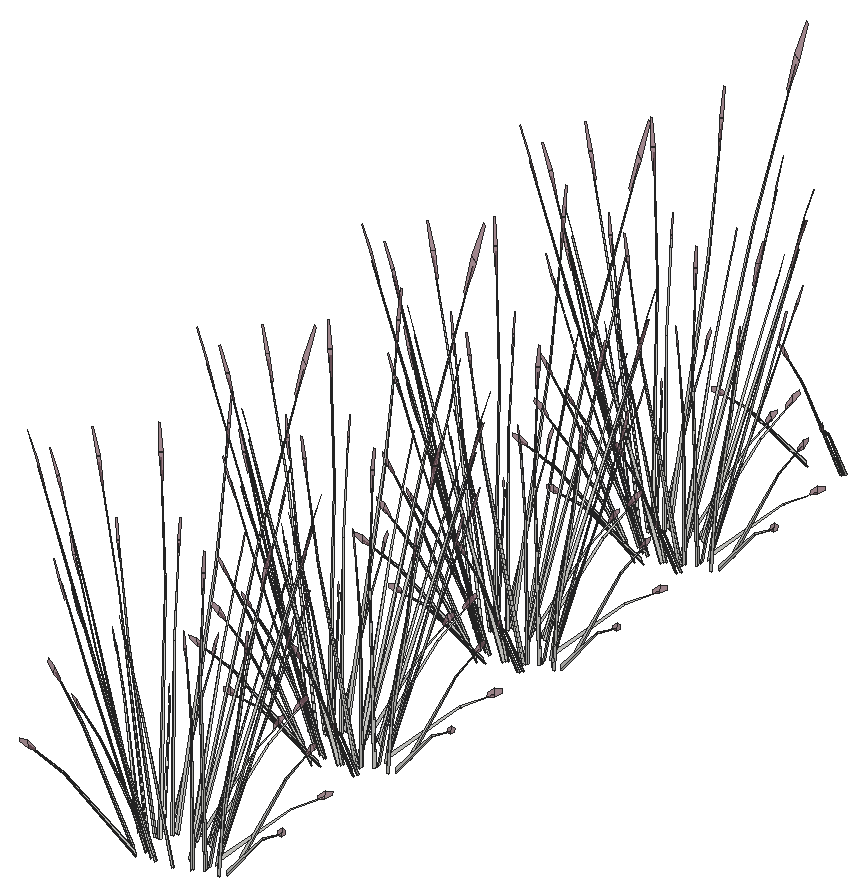
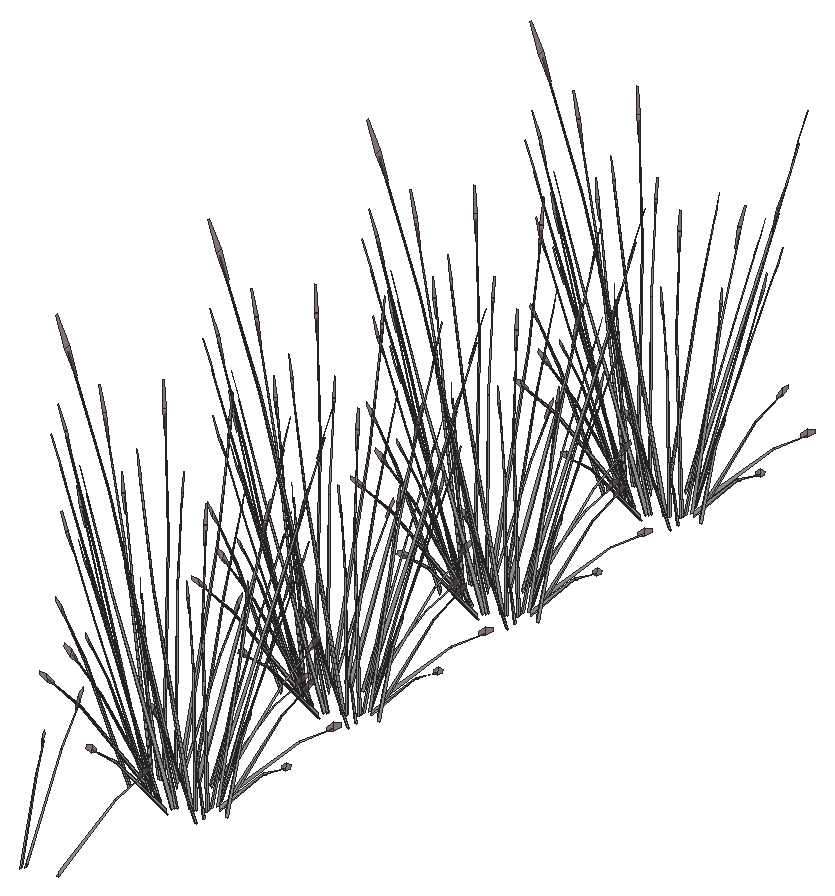
# SketchUp Ruby script. Lengths in inches.
U = 1.inch
M = Sketchup.active_model
def pt(a) = Geom::Point3d.new(a.map { |v| v * U })
def face(e, loops, mat)
  f = e.add_face(loops[0].map { |a| pt(a) })
  loops[1..].each { |l| e.add_face(l.map { |a| pt(a) }).erase! }
  f.material = f.back_material = mat if mat
  f
end
# faces: each face lists its corners as indices into pts; further lists are holes
def faces(e, pts, list, mat = nil) = list.each { |f| face(e, (f[0].is_a?(Array) ? f : [f]).map { |l| l.map { |i| pts[i] } }, mat) }
# xy, xz, yz: faces in a plane at the given z, y or x. An outline is a flat list of corners, or four numbers for a rectangle; further outlines are holes
def ring(l) = l.size == 4 ? [[l[0], l[1]], [l[2], l[1]], [l[2], l[3]], [l[0], l[3]]] : l.each_slice(2).to_a
def flat(e, list, mat, &to3) = list.each { |f| face(e, (f[0].is_a?(Array) ? f : [f]).map { |l| ring(l).map { |u, v| to3.(u, v) } }, mat) }
def xy(e, z, list, mat = nil) = flat(e, list, mat) { |x, y| [x, y, z] }
def xz(e, y, list, mat = nil) = flat(e, list, mat) { |x, z| [x, y, z] }
def yz(e, x, list, mat = nil) = flat(e, list, mat) { |y, z| [x, y, z] }
def lines(e, pts, list) = list.each { |a, b| e.add_line(pt(pts[a]), pt(pts[b])) }
# prism: a flat outline (further loops are holes) pulled along v
def prism(e, loops, v, mat = nil)
  f = face(e, loops, mat); d = Geom::Vector3d.new(v.map { |x| x * U })
  f.pushpull(f.normal.samedirection?(d) ? d.length : -d.length)
end
def box(e, o, s, mat = nil) = prism(e, [[o, [o[0] + s[0], o[1], o[2]], [o[0] + s[0], o[1] + s[1], o[2]], [o[0], o[1] + s[1], o[2]]]], [0, 0, s[2]], mat)
def at(x, y, z, deg = 0) = Geom::Transformation.translation(pt([x, y, z])) * Geom::Transformation.rotation(ORIGIN, Z_AXIS, deg.degrees)
def axes(o, x, y, z) = Geom::Transformation.new([*x, 0, *y, 0, *z, 0, *pt(o).to_a, 1])
def part(name) = M.definitions.add(name)
# library, detail: a bought-in or finely detailed component or shape, given as its bounding box
def library(name, o, s) = part(name).tap { |d| box(d.entities, o, s) }
def detail(e, o, s) = box(e.add_group.entities, o, s)
def put(e, d, t, mat = nil) = e.add_instance(d, t).tap { |i| i.material = mat if mat }
def group(e, t, mat = nil) = e.add_group.tap { |g| g.transformation = t; g.material = mat if mat }.entities
root = M.entities
M.materials.add("LightPink_Translucent").color = [144, 107, 117]
M.materials["LightPink_Translucent"].alpha = 0.75
c1 = part("blade")
p = [[2.15,0.21,22],[0,0.17,0],[0.09,0.45,0],[2.18,0.31,22],[2.29,0.31,22],[0.38,0.45,0],
  [2.48,0.24,33],[2.49,0.24,33],[2.48,0.22,33]]
faces(c1.entities,p,[[0,1,2,3],[4,5,2,3],[6,3,4,7],[8,0,3,6]])
c2 = part("seeds")
p = [[0.3,-0.1,1.38],[-0.01,-0.03,1.59],[-0.01,-0.03,0.03],[0.14,-0.07,-0.07],[0.29,-0.03,3],[0.15,0.01,3.11]]
faces(c2.entities,p,[[0,1,2,3],[1,0,4,5]],"LightPink_Translucent")
c3 = part("blade with seeds")
put(c3.entities,c1,at(0,0,0))
put(c3.entities,c2,axes([2.4,0.25,30.99],[1.5799,-0.05474,1.17369],[-0.12525,1.92788,0.29478],[-0.07173,-0.02425,1.56792]))
put(root,c3,axes([409.76,75.6,259.73],[0.55987,-0.20767,0.0643],[0.27403,0.37869,0.50621],[-0.05407,-0.16693,0.77189]))
put(root,c3,axes([407.84,75.65,259.73],[0.34533,-0.38816,0.0643],[0.49176,0.22599,0.50621],[-0.15898,-0.12445,0.77189]))
put(root,c3,axes([407.99,75.61,260.43],[-0.50709,0.58578,-0.13619],[-0.73436,-0.33748,-0.75594],[-0.25527,-0.1655,1.14864]))
put(root,c3,axes([411.46,76.26,259.73],[0.62439,0.02847,0.0643],[-0.01712,0.42991,0.50621],[0.06534,-0.16468,0.77189]))
put(root,c3,axes([406.05,75.45,259.72],[-0.16348,-0.00431,1.74944],[-0.52047,0.43131,-0.27667],[-0.2777,-0.08813,0.14031]))
put(root,c3,axes([412.23,77.59,260.03],[-0.70283,-0.33692,-0.1216],[0.40491,-0.48793,-0.67495],[0.19857,-0.16961,1.02557]))
put(root,c3,axes([413.96,77.45,259.71],[-0.09924,-0.00464,1.77383],[-0.4121,-0.49725,-0.16761],[0.1655,-0.1635,0.31391]))
put(root,c3,axes([406.22,76.42,259.73],[0.03826,-0.46465,0.0643],[0.57772,0.01274,0.50621],[-0.2213,-0.04862,0.77189]))
put(root,c3,axes([412.48,77.47,259.73],[0.52161,0.25698,0.0643],[-0.30368,0.36595,0.50621],[0.16723,-0.11831,0.77189]))
put(root,c3,axes([414.33,78.04,259.72],[0.10543,-0.09307,1.74944],[-0.13495,-0.57092,-0.27667],[0.26455,-0.10825,0.14031]))
put(root,c3,axes([405.42,75.8125,259.71],[0.05633,0.06098,1.77383],[-0.27155,0.54815,-0.16761],[-0.27501,0.00397,0.31391]))
put(root,c3,axes([406.49,76.52,260.03],[-0.04068,0.62141,-0.1216],[-0.77029,-0.01698,-0.67495],[-0.29667,-0.04317,1.02557]))
put(root,c3,axes([412.25,78.91,260.03],[-0.38229,-0.5533,-0.1216],[0.6785,-0.2719,-0.67495],[0.28593,-0.073,1.02557]))
put(root,c3,axes([405.32,77.68,259.73],[-0.27906,-0.41663,0.0643],[0.50888,-0.20393,0.50621],[-0.22432,0.04024,0.77189]))
put(root,c3,axes([412.5625,78.89,259.73],[0.27906,0.41663,0.0643],[-0.50888,0.20393,0.50621],[0.22432,-0.04024,0.77189]))
put(root,c3,axes([413.77,80.55,259.71],[-0.0687,-0.05349,1.77383],[0.15029,-0.57341,-0.16761],[0.27062,-0.03664,0.31391]))
put(root,c3,axes([404.83,78.22,259.72],[-0.12407,0.07933,1.74944],[0.01055,0.57963,-0.27667],[-0.2844,0.07538,0.14031]))
put(root,c3,axes([405.63,77.67,260.03],[0.38229,0.5533,-0.1216],[-0.6785,0.2719,-0.67495],[-0.28593,0.073,1.02557]))
put(root,c3,axes([411.4,80.06,260.03],[0.04068,-0.62141,-0.1216],[0.77029,0.01698,-0.67495],[0.29667,0.04317,1.02557]))
put(root,c3,axes([412.07,79.68,259.72],[0.16299,-0.01033,1.74944],[0.44707,-0.47471,-0.27667],[0.28992,0.06266,0.14031]))
put(root,c3,axes([405.4,79.11,259.73],[-0.52161,-0.25698,0.0643],[0.30368,-0.36595,0.50621],[-0.16723,0.11831,0.77189]))
put(root,c3,axes([403.45,78.81,259.71],[0.09697,0.01639,1.77383],[0.29997,0.53988,-0.16761],[-0.1985,0.1417,0.31391]))
put(root,c3,axes([411.67,80.16,259.73],[-0.03826,0.46465,0.0643],[-0.57772,-0.01274,0.50621],[0.2213,0.04862,0.77189]))
put(root,c3,axes([410.39,77.65,259.47],[-0.65655,-0.31748,1.38283],[0.69326,-0.49431,0.59665],[0.21183,0.29789,1.33663]))
put(root,c3,axes([405.66,78.99,260.03],[0.70283,0.33692,-0.1216],[-0.40491,0.48793,-0.67495],[-0.19857,0.16961,1.02557]))
put(root,c3,axes([409.88,80.73,260.03],[0.45276,-0.52302,-0.1216],[0.65568,0.30132,-0.67495],[0.22792,0.14777,1.02557]))
put(root,c3,axes([409.29,81.17,259.71],[0.00225,-0.07398,1.77383],[0.65113,-0.32638,-0.16761],[0.22617,0.1165,0.31391]))
put(root,c3,axes([406.43,80.32,259.73],[-0.62439,-0.02847,0.0643],[0.01712,-0.42991,0.50621],[-0.06534,0.16468,0.77189]))
put(root,c3,axes([410.05,80.92,259.73],[-0.34533,0.38816,0.0643],[-0.49176,-0.22599,0.50621],[0.15898,0.12445,0.77189]))
put(root,c3,axes([408.13,80.98,259.73],[-0.55987,0.20767,0.0643],[-0.27403,-0.37869,0.50621],[0.05407,0.16693,0.77189]))
put(root,c3,axes([404.85,80.39,259.72],[-0.01889,0.12092,1.74944],[0.53598,0.42065,-0.27667],[-0.14032,0.19892,0.14031]))
put(root,c3,axes([406.57,80.11,260.4],[0.83505,0.03027,-0.13498],[-0.02282,0.57322,-0.74919],[-0.05801,0.22077,1.13838]))
put(root,c3,axes([408.11,80.75,260.03],[0.74352,-0.28449,-0.1216],[0.36538,0.50492,-0.67495],[0.0981,0.21277,1.02557]))
put(root,c3,axes([404.79,81.63,259.71],[0.0862,-0.03689,1.77383],[0.71245,0.24539,-0.16761],[-0.01674,0.20431,0.31391]))
put(root,c3,axes([407.9375,81.88,259.72],[0.09631,0.0984,1.74944],[0.77725,0.03866,-0.27667],[0.07816,0.217,0.14031]))
put(root,c3,axes([408.72,98.03,259.72],[-0.11621,-0.08567,1.74944],[-0.77555,0.05431,-0.27667],[-0.12378,-0.20491,0.14031]))
put(root,c3,axes([412.2,99.08,259.72],[-0.00733,-0.12161,1.74944],[-0.61946,-0.35147,-0.27667],[0.09577,-0.21306,0.14031]))
put(root,c3,axes([412.04,98.64,259.71],[-0.07716,0.04667,1.77383],[-0.75601,-0.15746,-0.16761],[-0.02737,-0.20368,0.31391]))
put(root,c3,axes([407.92,97.75,259.71],[-0.01417,0.07324,1.77383],[-0.6991,0.2658,-0.16761],[-0.20573,-0.13587,0.31391]))
put(root,c3,axes([409.9,99.35,260.03],[-0.74352,0.28449,-0.1216],[-0.36538,-0.50492,-0.67495],[-0.0981,-0.21277,1.02557]))
put(root,c3,axes([411.44,99.99,260.03],[-0.83505,-0.03027,-0.1216],[0.02282,-0.57322,-0.67495],[0.05801,-0.22077,1.02557]))
put(root,c3,axes([409.88,99.12,259.73],[0.55987,-0.20767,0.0643],[0.27403,0.37869,0.50621],[-0.05407,-0.16693,0.77189]))
put(root,c3,axes([407.96,99.18,259.73],[0.34533,-0.38816,0.0643],[0.49176,0.22599,0.50621],[-0.15898,-0.12445,0.77189]))
put(root,c3,axes([408.12,99.14,260.43],[-0.50709,0.58578,-0.13619],[-0.73436,-0.33748,-0.75594],[-0.25527,-0.1655,1.14864]))
put(root,c3,axes([411.58,99.79,259.73],[0.62439,0.02847,0.0643],[-0.01712,0.42991,0.50621],[0.06534,-0.16468,0.77189]))
put(root,c3,axes([406.17,98.97,259.72],[-0.16348,-0.00431,1.74944],[-0.52047,0.43131,-0.27667],[-0.2777,-0.08813,0.14031]))
put(root,c3,axes([412.35,101.12,260.03],[-0.70283,-0.33692,-0.1216],[0.40491,-0.48793,-0.67495],[0.19857,-0.16961,1.02557]))
put(root,c3,axes([414.08,100.97,259.71],[-0.09924,-0.00464,1.77383],[-0.4121,-0.49725,-0.16761],[0.1655,-0.1635,0.31391]))
put(root,c3,axes([406.34,99.94,259.73],[0.03826,-0.46465,0.0643],[0.57772,0.01274,0.50621],[-0.2213,-0.04862,0.77189]))
put(root,c3,axes([412.61,100.99,259.73],[0.52161,0.25698,0.0643],[-0.30368,0.36595,0.50621],[0.16723,-0.11831,0.77189]))
put(root,c3,axes([414.46,101.57,259.72],[0.10543,-0.09307,1.74944],[-0.13495,-0.57092,-0.27667],[0.26455,-0.10825,0.14031]))
put(root,c3,axes([405.55,99.34,259.71],[0.05633,0.06098,1.77383],[-0.27155,0.54815,-0.16761],[-0.27501,0.00397,0.31391]))
put(root,c3,axes([406.61,100.05,260.03],[-0.04068,0.62141,-0.1216],[-0.77029,-0.01698,-0.67495],[-0.29667,-0.04317,1.02557]))
put(root,c3,axes([412.38,102.43,260.03],[-0.38229,-0.5533,-0.1216],[0.6785,-0.2719,-0.67495],[0.28593,-0.073,1.02557]))
put(root,c3,axes([405.45,101.21,259.73],[-0.27906,-0.41663,0.0643],[0.50888,-0.20393,0.50621],[-0.22432,0.04024,0.77189]))
put(root,c3,axes([412.6875,102.42,259.73],[0.27906,0.41663,0.0643],[-0.50888,0.20393,0.50621],[0.22432,-0.04024,0.77189]))
put(root,c3,axes([413.9,104.08,259.71],[-0.0687,-0.05349,1.77383],[0.15029,-0.57341,-0.16761],[0.27062,-0.03664,0.31391]))
put(root,c3,axes([404.96,101.75,259.72],[-0.12407,0.07933,1.74944],[0.01055,0.57963,-0.27667],[-0.2844,0.07538,0.14031]))
put(root,c3,axes([405.76,101.2,260.03],[0.38229,0.5533,-0.1216],[-0.6785,0.2719,-0.67495],[-0.28593,0.073,1.02557]))
put(root,c3,axes([411.52,103.58,260.03],[0.04068,-0.62141,-0.1216],[0.77029,0.01698,-0.67495],[0.29667,0.04317,1.02557]))
put(root,c3,axes([412.19,103.21,259.72],[0.16299,-0.01033,1.74944],[0.44707,-0.47471,-0.27667],[0.28992,0.06266,0.14031]))
put(root,c3,axes([405.53,102.64,259.73],[-0.52161,-0.25698,0.0643],[0.30368,-0.36595,0.50621],[-0.16723,0.11831,0.77189]))
put(root,c3,axes([403.58,102.34,259.71],[0.09697,0.01639,1.77383],[0.29997,0.53988,-0.16761],[-0.1985,0.1417,0.31391]))
put(root,c3,axes([411.79,103.6875,259.73],[-0.03826,0.46465,0.0643],[-0.57772,-0.01274,0.50621],[0.2213,0.04862,0.77189]))
put(root,c3,axes([410.52,101.17,259.47],[-0.65655,-0.31748,1.38283],[0.69326,-0.49431,0.59665],[0.21183,0.29789,1.33663]))
put(root,c3,axes([405.78,102.51,260.03],[0.70283,0.33692,-0.1216],[-0.40491,0.48793,-0.67495],[-0.19857,0.16961,1.02557]))
put(root,c3,axes([410,104.26,260.03],[0.45276,-0.52302,-0.1216],[0.65568,0.30132,-0.67495],[0.22792,0.14777,1.02557]))
put(root,c3,axes([409.41,104.69,259.71],[0.00225,-0.07398,1.77383],[0.65113,-0.32638,-0.16761],[0.22617,0.1165,0.31391]))
put(root,c3,axes([406.55,103.84,259.73],[-0.62439,-0.02847,0.0643],[0.01712,-0.42991,0.50621],[-0.06534,0.16468,0.77189]))
put(root,c3,axes([410.17,104.45,259.73],[-0.34533,0.38816,0.0643],[-0.49176,-0.22599,0.50621],[0.15898,0.12445,0.77189]))
put(root,c3,axes([408.25,104.51,259.73],[-0.55987,0.20767,0.0643],[-0.27403,-0.37869,0.50621],[0.05407,0.16693,0.77189]))
put(root,c3,axes([404.98,103.91,259.72],[-0.01889,0.12092,1.74944],[0.53598,0.42065,-0.27667],[-0.14032,0.19892,0.14031]))
put(root,c3,axes([406.69,103.64,260.4],[0.83505,0.03027,-0.13498],[-0.02282,0.57322,-0.74919],[-0.05801,0.22077,1.13838]))
put(root,c3,axes([408.24,104.28,260.03],[0.74352,-0.28449,-0.1216],[0.36538,0.50492,-0.67495],[0.0981,0.21277,1.02557]))
put(root,c3,axes([404.92,105.15,259.71],[0.0862,-0.03689,1.77383],[0.71245,0.24539,-0.16761],[-0.01674,0.20431,0.31391]))
put(root,c3,axes([408.0625,105.41,259.72],[0.09631,0.0984,1.74944],[0.77725,0.03866,-0.27667],[0.07816,0.217,0.14031]))
put(root,c3,axes([408.5,121.42,259.72],[-0.11621,-0.08567,1.74944],[-0.77555,0.05431,-0.27667],[-0.12378,-0.20491,0.14031]))
put(root,c3,axes([411.98,122.47,259.72],[-0.00733,-0.12161,1.74944],[-0.61946,-0.35147,-0.27667],[0.09577,-0.21306,0.14031]))
put(root,c3,axes([411.82,122.03,259.71],[-0.07716,0.04667,1.77383],[-0.75601,-0.15746,-0.16761],[-0.02737,-0.20368,0.31391]))
put(root,c3,axes([407.7,121.13,259.71],[-0.01417,0.07324,1.77383],[-0.6991,0.2658,-0.16761],[-0.20573,-0.13587,0.31391]))
put(root,c3,axes([409.68,122.74,260.03],[-0.74352,0.28449,-0.1216],[-0.36538,-0.50492,-0.67495],[-0.0981,-0.21277,1.02557]))
put(root,c3,axes([411.22,123.375,260.03],[-0.83505,-0.03027,-0.1216],[0.02282,-0.57322,-0.67495],[0.05801,-0.22077,1.02557]))
put(root,c3,axes([409.66,122.51,259.73],[0.55987,-0.20767,0.0643],[0.27403,0.37869,0.50621],[-0.05407,-0.16693,0.77189]))
put(root,c3,axes([407.74,122.57,259.73],[0.34533,-0.38816,0.0643],[0.49176,0.22599,0.50621],[-0.15898,-0.12445,0.77189]))
put(root,c3,axes([407.9,122.53,260.43],[-0.50709,0.58578,-0.13619],[-0.73436,-0.33748,-0.75594],[-0.25527,-0.1655,1.14864]))
put(root,c3,axes([411.36,123.17,259.73],[0.62439,0.02847,0.0643],[-0.01712,0.42991,0.50621],[0.06534,-0.16468,0.77189]))
put(root,c3,axes([405.96,122.36,259.72],[-0.16348,-0.00431,1.74944],[-0.52047,0.43131,-0.27667],[-0.2777,-0.08813,0.14031]))
put(root,c3,axes([412.13,124.5,260.03],[-0.70283,-0.33692,-0.1216],[0.40491,-0.48793,-0.67495],[0.19857,-0.16961,1.02557]))
put(root,c3,axes([413.86,124.36,259.71],[-0.09924,-0.00464,1.77383],[-0.4121,-0.49725,-0.16761],[0.1655,-0.1635,0.31391]))
put(root,c3,axes([406.12,123.33,259.73],[0.03826,-0.46465,0.0643],[0.57772,0.01274,0.50621],[-0.2213,-0.04862,0.77189]))
put(root,c3,axes([412.39,124.38,259.73],[0.52161,0.25698,0.0643],[-0.30368,0.36595,0.50621],[0.16723,-0.11831,0.77189]))
put(root,c3,axes([414.24,124.95,259.72],[0.10543,-0.09307,1.74944],[-0.13495,-0.57092,-0.27667],[0.26455,-0.10825,0.14031]))
put(root,c3,axes([405.33,122.72,259.71],[0.05633,0.06098,1.77383],[-0.27155,0.54815,-0.16761],[-0.27501,0.00397,0.31391]))
put(root,c3,axes([406.4,123.43,260.03],[-0.04068,0.62141,-0.1216],[-0.77029,-0.01698,-0.67495],[-0.29667,-0.04317,1.02557]))
put(root,c3,axes([412.16,125.82,260.03],[-0.38229,-0.5533,-0.1216],[0.6785,-0.2719,-0.67495],[0.28593,-0.073,1.02557]))
put(root,c3,axes([405.23,124.6,259.73],[-0.27906,-0.41663,0.0643],[0.50888,-0.20393,0.50621],[-0.22432,0.04024,0.77189]))
put(root,c3,axes([412.47,125.81,259.73],[0.27906,0.41663,0.0643],[-0.50888,0.20393,0.50621],[0.22432,-0.04024,0.77189]))
put(root,c3,axes([413.68,127.46,259.71],[-0.0687,-0.05349,1.77383],[0.15029,-0.57341,-0.16761],[0.27062,-0.03664,0.31391]))
put(root,c3,axes([404.74,125.14,259.72],[-0.12407,0.07933,1.74944],[0.01055,0.57963,-0.27667],[-0.2844,0.07538,0.14031]))
put(root,c3,axes([405.54,124.58,260.03],[0.38229,0.5533,-0.1216],[-0.6785,0.2719,-0.67495],[-0.28593,0.073,1.02557]))
put(root,c3,axes([411.3,126.97,260.03],[0.04068,-0.62141,-0.1216],[0.77029,0.01698,-0.67495],[0.29667,0.04317,1.02557]))
put(root,c3,axes([411.97,126.6,259.72],[0.16299,-0.01033,1.74944],[0.44707,-0.47471,-0.27667],[0.28992,0.06266,0.14031]))
put(root,c3,axes([405.31,126.02,259.73],[-0.52161,-0.25698,0.0643],[0.30368,-0.36595,0.50621],[-0.16723,0.11831,0.77189]))
put(root,c3,axes([403.36,125.72,259.71],[0.09697,0.01639,1.77383],[0.29997,0.53988,-0.16761],[-0.1985,0.1417,0.31391]))
put(root,c3,axes([411.58,127.07,259.73],[-0.03826,0.46465,0.0643],[-0.57772,-0.01274,0.50621],[0.2213,0.04862,0.77189]))
put(root,c3,axes([410.3,124.56,259.47],[-0.65655,-0.31748,1.38283],[0.69326,-0.49431,0.59665],[0.21183,0.29789,1.33663]))
put(root,c3,axes([405.57,125.9,260.03],[0.70283,0.33692,-0.1216],[-0.40491,0.48793,-0.67495],[-0.19857,0.16961,1.02557]))
put(root,c3,axes([409.79,127.65,260.03],[0.45276,-0.52302,-0.1216],[0.65568,0.30132,-0.67495],[0.22792,0.14777,1.02557]))
put(root,c3,axes([409.19,128.08,259.71],[0.00225,-0.07398,1.77383],[0.65113,-0.32638,-0.16761],[0.22617,0.1165,0.31391]))
put(root,c3,axes([406.34,127.23,259.73],[-0.62439,-0.02847,0.0643],[0.01712,-0.42991,0.50621],[-0.06534,0.16468,0.77189]))
put(root,c3,axes([409.95,127.84,259.73],[-0.34533,0.38816,0.0643],[-0.49176,-0.22599,0.50621],[0.15898,0.12445,0.77189]))
put(root,c3,axes([408.04,127.89,259.73],[-0.55987,0.20767,0.0643],[-0.27403,-0.37869,0.50621],[0.05407,0.16693,0.77189]))
put(root,c3,axes([404.76,127.3,259.72],[-0.01889,0.12092,1.74944],[0.53598,0.42065,-0.27667],[-0.14032,0.19892,0.14031]))
put(root,c3,axes([406.47,127.03,260.4],[0.83505,0.03027,-0.13498],[-0.02282,0.57322,-0.74919],[-0.05801,0.22077,1.13838]))
put(root,c3,axes([408.02,127.67,260.03],[0.74352,-0.28449,-0.1216],[0.36538,0.50492,-0.67495],[0.0981,0.21277,1.02557]))
put(root,c3,axes([404.7,128.54,259.71],[0.0862,-0.03689,1.77383],[0.71245,0.24539,-0.16761],[-0.01674,0.20431,0.31391]))
put(root,c3,axes([407.84,128.8,259.72],[0.09631,0.0984,1.74944],[0.77725,0.03866,-0.27667],[0.07816,0.217,0.14031]))
put(root,c3,axes([408.22,143.83,259.72],[-0.11621,-0.08567,1.74944],[-0.77555,0.05431,-0.27667],[-0.12378,-0.20491,0.14031]))
put(root,c3,axes([411.7,144.875,259.72],[-0.00733,-0.12161,1.74944],[-0.61946,-0.35147,-0.27667],[0.09577,-0.21306,0.14031]))
put(root,c3,axes([411.54,144.4375,259.71],[-0.07716,0.04667,1.77383],[-0.75601,-0.15746,-0.16761],[-0.02737,-0.20368,0.31391]))
put(root,c3,axes([407.43,143.54,259.71],[-0.01417,0.07324,1.77383],[-0.6991,0.2658,-0.16761],[-0.20573,-0.13587,0.31391]))
put(root,c3,axes([409.4,145.15,260.03],[-0.74352,0.28449,-0.1216],[-0.36538,-0.50492,-0.67495],[-0.0981,-0.21277,1.02557]))
put(root,c3,axes([410.95,145.79,260.03],[-0.83505,-0.03027,-0.1216],[0.02282,-0.57322,-0.67495],[0.05801,-0.22077,1.02557]))
put(root,c3,axes([409.38,144.92,259.73],[0.55987,-0.20767,0.0643],[0.27403,0.37869,0.50621],[-0.05407,-0.16693,0.77189]))
put(root,c3,axes([407.47,144.98,259.73],[0.34533,-0.38816,0.0643],[0.49176,0.22599,0.50621],[-0.15898,-0.12445,0.77189]))
put(root,c3,axes([407.62,144.9375,260.43],[-0.50709,0.58578,-0.13619],[-0.73436,-0.33748,-0.75594],[-0.25527,-0.1655,1.14864]))
put(root,c3,axes([411.08,145.58,259.73],[0.62439,0.02847,0.0643],[-0.01712,0.42991,0.50621],[0.06534,-0.16468,0.77189]))
put(root,c3,axes([405.68,144.77,259.72],[-0.16348,-0.00431,1.74944],[-0.52047,0.43131,-0.27667],[-0.2777,-0.08813,0.14031]))
put(root,c3,axes([411.85,146.91,260.03],[-0.70283,-0.33692,-0.1216],[0.40491,-0.48793,-0.67495],[0.19857,-0.16961,1.02557]))
put(root,c3,axes([413.58,146.77,259.71],[-0.09924,-0.00464,1.77383],[-0.4121,-0.49725,-0.16761],[0.1655,-0.1635,0.31391]))
put(root,c3,axes([405.84,145.74,259.73],[0.03826,-0.46465,0.0643],[0.57772,0.01274,0.50621],[-0.2213,-0.04862,0.77189]))
put(root,c3,axes([412.11,146.79,259.73],[0.52161,0.25698,0.0643],[-0.30368,0.36595,0.50621],[0.16723,-0.11831,0.77189]))
put(root,c3,axes([413.96,147.36,259.72],[0.10543,-0.09307,1.74944],[-0.13495,-0.57092,-0.27667],[0.26455,-0.10825,0.14031]))
put(root,c3,axes([405.05,145.13,259.71],[0.05633,0.06098,1.77383],[-0.27155,0.54815,-0.16761],[-0.27501,0.00397,0.31391]))
put(root,c3,axes([406.12,145.84,260.03],[-0.04068,0.62141,-0.1216],[-0.77029,-0.01698,-0.67495],[-0.29667,-0.04317,1.02557]))
put(root,c3,axes([411.88,148.23,260.03],[-0.38229,-0.5533,-0.1216],[0.6785,-0.2719,-0.67495],[0.28593,-0.073,1.02557]))
put(root,c3,axes([404.95,147.01,259.73],[-0.27906,-0.41663,0.0643],[0.50888,-0.20393,0.50621],[-0.22432,0.04024,0.77189]))
put(root,c3,axes([412.1875,148.22,259.73],[0.27906,0.41663,0.0643],[-0.50888,0.20393,0.50621],[0.22432,-0.04024,0.77189]))
put(root,c3,axes([413.4,149.875,259.71],[-0.0687,-0.05349,1.77383],[0.15029,-0.57341,-0.16761],[0.27062,-0.03664,0.31391]))
put(root,c3,axes([404.46,147.55,259.72],[-0.12407,0.07933,1.74944],[0.01055,0.57963,-0.27667],[-0.2844,0.07538,0.14031]))
put(root,c3,axes([405.26,146.99,260.03],[0.38229,0.5533,-0.1216],[-0.6785,0.2719,-0.67495],[-0.28593,0.073,1.02557]))
put(root,c3,axes([411.02,149.38,260.03],[0.04068,-0.62141,-0.1216],[0.77029,0.01698,-0.67495],[0.29667,0.04317,1.02557]))
put(root,c3,axes([411.69,149.01,259.72],[0.16299,-0.01033,1.74944],[0.44707,-0.47471,-0.27667],[0.28992,0.06266,0.14031]))
put(root,c3,axes([405.03,148.43,259.73],[-0.52161,-0.25698,0.0643],[0.30368,-0.36595,0.50621],[-0.16723,0.11831,0.77189]))
put(root,c3,axes([403.08,148.13,259.71],[0.09697,0.01639,1.77383],[0.29997,0.53988,-0.16761],[-0.1985,0.1417,0.31391]))
put(root,c3,axes([411.3,149.48,259.73],[-0.03826,0.46465,0.0643],[-0.57772,-0.01274,0.50621],[0.2213,0.04862,0.77189]))
put(root,c3,axes([410.02,146.97,259.47],[-0.65655,-0.31748,1.38283],[0.69326,-0.49431,0.59665],[0.21183,0.29789,1.33663]))
put(root,c3,axes([405.29,148.31,260.03],[0.70283,0.33692,-0.1216],[-0.40491,0.48793,-0.67495],[-0.19857,0.16961,1.02557]))
put(root,c3,axes([409.51,150.06,260.03],[0.45276,-0.52302,-0.1216],[0.65568,0.30132,-0.67495],[0.22792,0.14777,1.02557]))
put(root,c3,axes([408.91,150.49,259.71],[0.00225,-0.07398,1.77383],[0.65113,-0.32638,-0.16761],[0.22617,0.1165,0.31391]))
put(root,c3,axes([406.06,149.64,259.73],[-0.62439,-0.02847,0.0643],[0.01712,-0.42991,0.50621],[-0.06534,0.16468,0.77189]))
put(root,c3,axes([409.68,150.25,259.73],[-0.34533,0.38816,0.0643],[-0.49176,-0.22599,0.50621],[0.15898,0.12445,0.77189]))
put(root,c3,axes([407.76,150.3,259.73],[-0.55987,0.20767,0.0643],[-0.27403,-0.37869,0.50621],[0.05407,0.16693,0.77189]))
put(root,c3,axes([404.48,149.71,259.72],[-0.01889,0.12092,1.74944],[0.53598,0.42065,-0.27667],[-0.14032,0.19892,0.14031]))
put(root,c3,axes([406.2,149.4375,260.4],[0.83505,0.03027,-0.13498],[-0.02282,0.57322,-0.74919],[-0.05801,0.22077,1.13838]))
put(root,c3,axes([407.74,150.08,260.03],[0.74352,-0.28449,-0.1216],[0.36538,0.50492,-0.67495],[0.0981,0.21277,1.02557]))
put(root,c3,axes([404.42,150.95,259.71],[0.0862,-0.03689,1.77383],[0.71245,0.24539,-0.16761],[-0.01674,0.20431,0.31391]))
put(root,c3,axes([407.57,151.21,259.72],[0.09631,0.0984,1.74944],[0.77725,0.03866,-0.27667],[0.07816,0.217,0.14031]))
put(root,c3,axes([408.58,166.42,259.72],[-0.11621,-0.08567,1.74944],[-0.77555,0.05431,-0.27667],[-0.12378,-0.20491,0.14031]))
put(root,c3,axes([412.07,167.47,259.72],[-0.00733,-0.12161,1.74944],[-0.61946,-0.35147,-0.27667],[0.09577,-0.21306,0.14031]))
put(root,c3,axes([411.9,167.03,259.71],[-0.07716,0.04667,1.77383],[-0.75601,-0.15746,-0.16761],[-0.02737,-0.20368,0.31391]))
